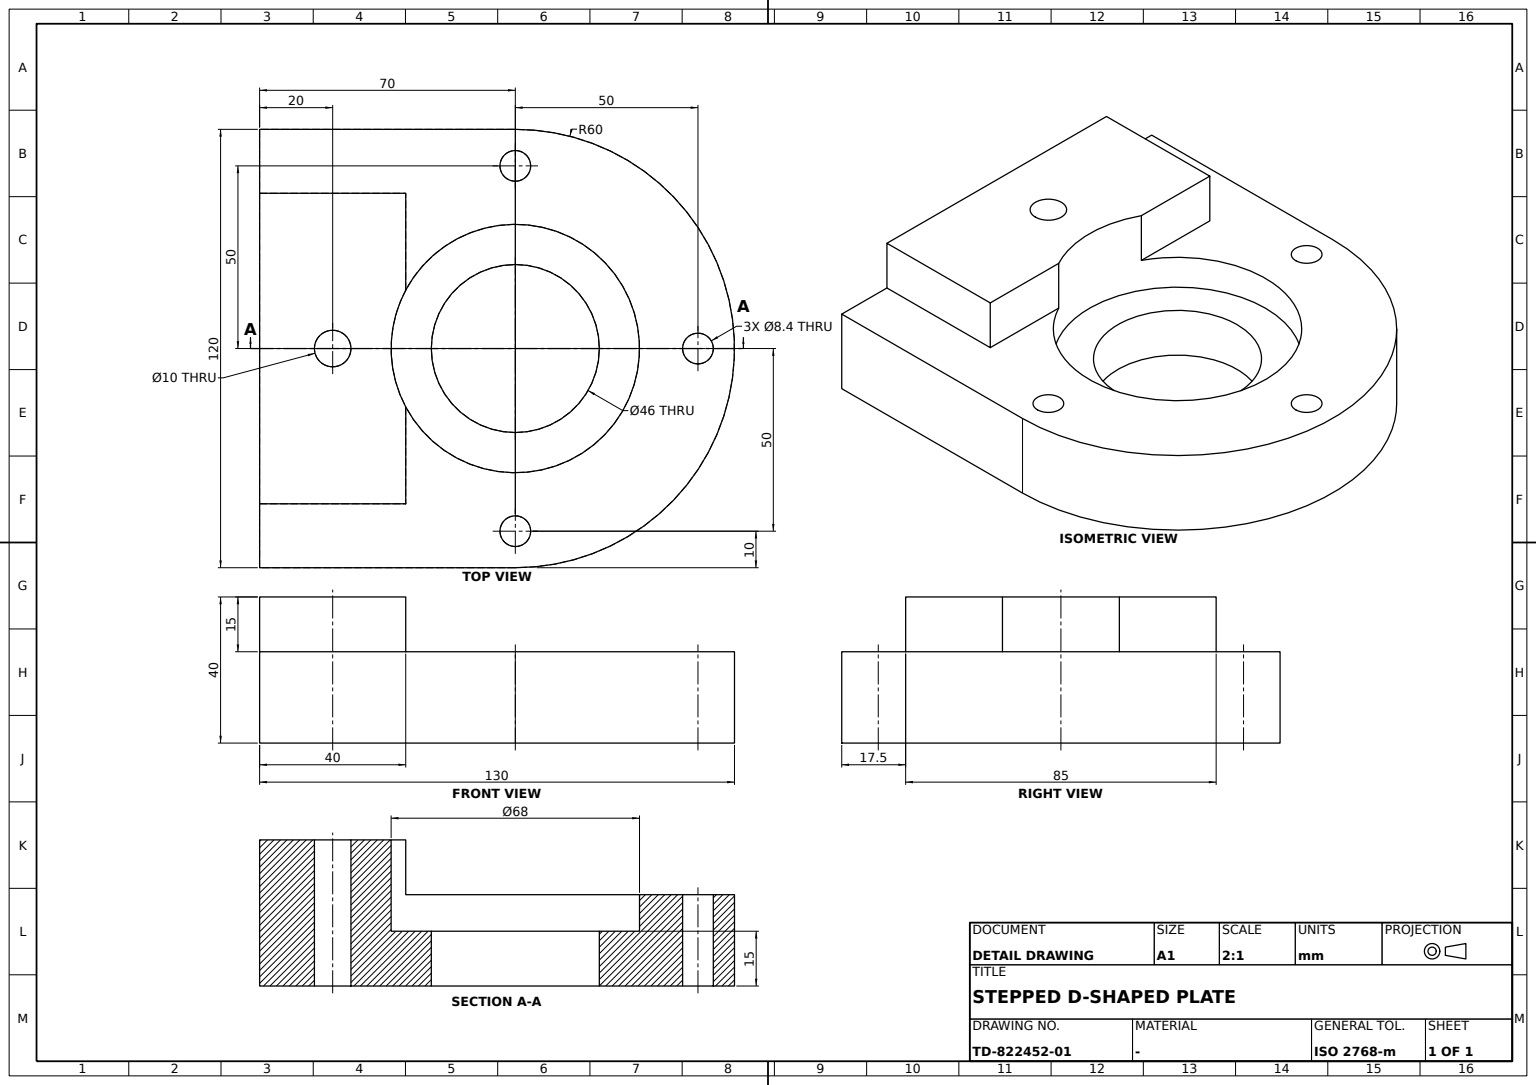
ISO-10303-21;
HEADER;
FILE_DESCRIPTION((''),'2;1');
FILE_NAME('','',(''),(''),'','','');
FILE_SCHEMA(('AUTOMOTIVE_DESIGN'));
ENDSEC;
DATA;
#1=APPLICATION_CONTEXT('');
#2=PRODUCT_CONTEXT('',#1,'mechanical');
#3=PRODUCT('','','',(#2));
#4=PRODUCT_DEFINITION_FORMATION('','',#3);
#5=PRODUCT_DEFINITION_CONTEXT('',#1,'design');
#6=PRODUCT_DEFINITION('','',#4,#5);
#7=PRODUCT_DEFINITION_SHAPE('','',#6);
#8=(LENGTH_UNIT()NAMED_UNIT(*)SI_UNIT(.MILLI.,.METRE.));
#9=(NAMED_UNIT(*)PLANE_ANGLE_UNIT()SI_UNIT($,.RADIAN.));
#10=(NAMED_UNIT(*)SI_UNIT($,.STERADIAN.)SOLID_ANGLE_UNIT());
#11=UNCERTAINTY_MEASURE_WITH_UNIT(LENGTH_MEASURE(0.005),#8,'distance_accuracy_value','');
#12=(GEOMETRIC_REPRESENTATION_CONTEXT(3)GLOBAL_UNCERTAINTY_ASSIGNED_CONTEXT((#11))GLOBAL_UNIT_ASSIGNED_CONTEXT((#8,#9,#10))REPRESENTATION_CONTEXT('',''));
#13=CARTESIAN_POINT('',(-45.797717,0.,25.));
#14=VERTEX_POINT('',#13);
#15=CARTESIAN_POINT('',(-50.,0.,25.));
#16=DIRECTION('',(0.,0.,1.));
#17=DIRECTION('',(1.,0.,0.));
#18=AXIS2_PLACEMENT_3D('',#15,#16,#17);
#19=CIRCLE('',#18,4.202283);
#20=EDGE_CURVE('',#14,#14,#19,.T.);
#21=ORIENTED_EDGE('',*,*,#20,.T.);
#22=EDGE_LOOP('',(#21));
#23=FACE_BOUND('',#22,.T.);
#24=CARTESIAN_POINT('',(-45.797717,0.,0.));
#25=VERTEX_POINT('',#24);
#26=CARTESIAN_POINT('',(-50.,0.,0.));
#27=AXIS2_PLACEMENT_3D('',#26,#16,#17);
#28=CIRCLE('',#27,4.202283);
#29=EDGE_CURVE('',#25,#25,#28,.T.);
#30=ORIENTED_EDGE('',*,*,#29,.F.);
#31=EDGE_LOOP('',(#30));
#32=FACE_BOUND('',#31,.T.);
#33=CARTESIAN_POINT('',(-50.,0.,11.84));
#34=DIRECTION('',(0.,1.,0.));
#35=AXIS2_PLACEMENT_3D('',#33,#16,#34);
#36=CYLINDRICAL_SURFACE('',#35,4.202283);
#37=ADVANCED_FACE('',(#23,#32),#36,.F.);
#38=CARTESIAN_POINT('',(-16.,-30.,25.));
#39=VERTEX_POINT('',#38);
#40=CARTESIAN_POINT('',(-16.,-30.,40.));
#41=VERTEX_POINT('',#40);
#42=DIRECTION('',(0.,0.,-1.));
#43=VECTOR('',#42,1000.);
#44=LINE('',#38,#43);
#45=EDGE_CURVE('',#39,#41,#44,.F.);
#46=ORIENTED_EDGE('',*,*,#45,.F.);
#47=CARTESIAN_POINT('',(-42.5,-30.,25.));
#48=VERTEX_POINT('',#47);
#49=CARTESIAN_POINT('',(0.,-30.,25.));
#50=DIRECTION('',(-1.,0.,0.));
#51=VECTOR('',#50,1000.);
#52=LINE('',#49,#51);
#53=EDGE_CURVE('',#39,#48,#52,.T.);
#54=ORIENTED_EDGE('',*,*,#53,.T.);
#55=CARTESIAN_POINT('',(-42.5,-30.,40.));
#56=VERTEX_POINT('',#55);
#57=VECTOR('',#16,1000.);
#58=LINE('',#47,#57);
#59=EDGE_CURVE('',#48,#56,#58,.T.);
#60=ORIENTED_EDGE('',*,*,#59,.T.);
#61=CARTESIAN_POINT('',(0.,-30.,40.));
#62=LINE('',#61,#51);
#63=EDGE_CURVE('',#41,#56,#62,.T.);
#64=ORIENTED_EDGE('',*,*,#63,.F.);
#65=EDGE_LOOP('',(#46,#54,#60,#64));
#66=FACE_BOUND('',#65,.T.);
#67=CARTESIAN_POINT('',(42.5,-30.,25.));
#68=AXIS2_PLACEMENT_3D('',#67,#34,#50);
#69=PLANE('',#68);
#70=ADVANCED_FACE('',(#66),#69,.T.);
#71=CARTESIAN_POINT('',(-34.,0.,15.));
#72=VERTEX_POINT('',#71);
#73=CARTESIAN_POINT('',(0.,0.,15.));
#74=AXIS2_PLACEMENT_3D('',#73,#42,#50);
#75=CIRCLE('',#74,34.);
#76=EDGE_CURVE('',#72,#72,#75,.T.);
#77=ORIENTED_EDGE('',*,*,#76,.F.);
#78=EDGE_LOOP('',(#77));
#79=FACE_BOUND('',#78,.T.);
#80=CARTESIAN_POINT('',(-23.,0.,15.));
#81=VERTEX_POINT('',#80);
#82=CIRCLE('',#74,23.);
#83=EDGE_CURVE('',#81,#81,#82,.T.);
#84=ORIENTED_EDGE('',*,*,#83,.T.);
#85=EDGE_LOOP('',(#84));
#86=FACE_BOUND('',#85,.T.);
#87=AXIS2_PLACEMENT_3D('',#73,#42,#17);
#88=PLANE('',#87);
#89=ADVANCED_FACE('',(#79,#86),#88,.F.);
#90=CARTESIAN_POINT('',(-60.,0.,0.));
#91=VERTEX_POINT('',#90);
#92=CARTESIAN_POINT('',(-60.,0.,25.));
#93=VERTEX_POINT('',#92);
#94=CARTESIAN_POINT('',(-60.,0.,12.5));
#95=LINE('',#94,#57);
#96=EDGE_CURVE('',#91,#93,#95,.T.);
#97=ORIENTED_EDGE('',*,*,#96,.T.);
#98=CARTESIAN_POINT('',(60.,0.,25.));
#99=VERTEX_POINT('',#98);
#100=CARTESIAN_POINT('',(0.,0.,25.));
#101=AXIS2_PLACEMENT_3D('',#100,#16,#17);
#102=CIRCLE('',#101,60.);
#103=EDGE_CURVE('',#99,#93,#102,.T.);
#104=ORIENTED_EDGE('',*,*,#103,.F.);
#105=CARTESIAN_POINT('',(60.,0.,0.));
#106=VERTEX_POINT('',#105);
#107=CARTESIAN_POINT('',(60.,0.,12.5));
#108=LINE('',#107,#57);
#109=EDGE_CURVE('',#106,#99,#108,.T.);
#110=ORIENTED_EDGE('',*,*,#109,.F.);
#111=CARTESIAN_POINT('',(0.,0.,0.));
#112=AXIS2_PLACEMENT_3D('',#111,#16,#17);
#113=CIRCLE('',#112,60.);
#114=EDGE_CURVE('',#106,#91,#113,.T.);
#115=ORIENTED_EDGE('',*,*,#114,.T.);
#116=EDGE_LOOP('',(#97,#104,#110,#115));
#117=FACE_BOUND('',#116,.T.);
#118=CARTESIAN_POINT('',(0.,0.,12.5));
#119=AXIS2_PLACEMENT_3D('',#118,#16,#34);
#120=CYLINDRICAL_SURFACE('',#119,60.);
#121=ADVANCED_FACE('',(#117),#120,.T.);
#122=CARTESIAN_POINT('',(-60.,-70.,0.));
#123=VERTEX_POINT('',#122);
#124=CARTESIAN_POINT('',(-60.,-70.,25.));
#125=VERTEX_POINT('',#124);
#126=LINE('',#122,#57);
#127=EDGE_CURVE('',#123,#125,#126,.T.);
#128=ORIENTED_EDGE('',*,*,#127,.T.);
#129=DIRECTION('',(0.,-1.,0.));
#130=VECTOR('',#129,1000.);
#131=LINE('',#92,#130);
#132=EDGE_CURVE('',#93,#125,#131,.T.);
#133=ORIENTED_EDGE('',*,*,#132,.F.);
#134=ORIENTED_EDGE('',*,*,#96,.F.);
#135=LINE('',#90,#130);
#136=EDGE_CURVE('',#91,#123,#135,.T.);
#137=ORIENTED_EDGE('',*,*,#136,.T.);
#138=EDGE_LOOP('',(#128,#133,#134,#137));
#139=FACE_BOUND('',#138,.T.);
#140=AXIS2_PLACEMENT_3D('',#90,#50,#129);
#141=PLANE('',#140);
#142=ADVANCED_FACE('',(#139),#141,.T.);
#143=CARTESIAN_POINT('',(-42.5,-70.,25.));
#144=VERTEX_POINT('',#143);
#145=CARTESIAN_POINT('',(0.,-70.,25.));
#146=VECTOR('',#17,1000.);
#147=LINE('',#145,#146);
#148=EDGE_CURVE('',#125,#144,#147,.T.);
#149=ORIENTED_EDGE('',*,*,#148,.F.);
#150=ORIENTED_EDGE('',*,*,#127,.F.);
#151=CARTESIAN_POINT('',(60.,-70.,0.));
#152=VERTEX_POINT('',#151);
#153=CARTESIAN_POINT('',(0.,-70.,0.));
#154=LINE('',#153,#146);
#155=EDGE_CURVE('',#123,#152,#154,.T.);
#156=ORIENTED_EDGE('',*,*,#155,.T.);
#157=CARTESIAN_POINT('',(60.,-70.,25.));
#158=VERTEX_POINT('',#157);
#159=LINE('',#151,#57);
#160=EDGE_CURVE('',#152,#158,#159,.T.);
#161=ORIENTED_EDGE('',*,*,#160,.T.);
#162=CARTESIAN_POINT('',(42.5,-70.,25.));
#163=VERTEX_POINT('',#162);
#164=EDGE_CURVE('',#163,#158,#147,.T.);
#165=ORIENTED_EDGE('',*,*,#164,.F.);
#166=CARTESIAN_POINT('',(42.5,-70.,40.));
#167=VERTEX_POINT('',#166);
#168=LINE('',#162,#57);
#169=EDGE_CURVE('',#163,#167,#168,.T.);
#170=ORIENTED_EDGE('',*,*,#169,.T.);
#171=CARTESIAN_POINT('',(-42.5,-70.,40.));
#172=VERTEX_POINT('',#171);
#173=CARTESIAN_POINT('',(0.,-70.,40.));
#174=LINE('',#173,#146);
#175=EDGE_CURVE('',#172,#167,#174,.T.);
#176=ORIENTED_EDGE('',*,*,#175,.F.);
#177=CARTESIAN_POINT('',(-42.5,-70.,0.));
#178=LINE('',#177,#57);
#179=EDGE_CURVE('',#144,#172,#178,.T.);
#180=ORIENTED_EDGE('',*,*,#179,.F.);
#181=EDGE_LOOP('',(#149,#150,#156,#161,#165,#170,#176,#180));
#182=FACE_BOUND('',#181,.T.);
#183=AXIS2_PLACEMENT_3D('',#122,#129,#17);
#184=PLANE('',#183);
#185=ADVANCED_FACE('',(#182),#184,.T.);
#186=ORIENTED_EDGE('',*,*,#169,.F.);
#187=VERTEX_POINT('',#67);
#188=CARTESIAN_POINT('',(42.5,0.,25.));
#189=LINE('',#188,#130);
#190=EDGE_CURVE('',#187,#163,#189,.T.);
#191=ORIENTED_EDGE('',*,*,#190,.F.);
#192=CARTESIAN_POINT('',(42.5,-30.,40.));
#193=VERTEX_POINT('',#192);
#194=LINE('',#67,#57);
#195=EDGE_CURVE('',#187,#193,#194,.T.);
#196=ORIENTED_EDGE('',*,*,#195,.T.);
#197=CARTESIAN_POINT('',(42.5,0.,40.));
#198=LINE('',#197,#130);
#199=EDGE_CURVE('',#193,#167,#198,.T.);
#200=ORIENTED_EDGE('',*,*,#199,.T.);
#201=EDGE_LOOP('',(#186,#191,#196,#200));
#202=FACE_BOUND('',#201,.T.);
#203=AXIS2_PLACEMENT_3D('',#67,#50,#129);
#204=PLANE('',#203);
#205=ADVANCED_FACE('',(#202),#204,.F.);
#206=CARTESIAN_POINT('',(4.202283,50.,25.));
#207=VERTEX_POINT('',#206);
#208=CARTESIAN_POINT('',(0.,50.,25.));
#209=AXIS2_PLACEMENT_3D('',#208,#16,#17);
#210=CIRCLE('',#209,4.202283);
#211=EDGE_CURVE('',#207,#207,#210,.T.);
#212=ORIENTED_EDGE('',*,*,#211,.F.);
#213=EDGE_LOOP('',(#212));
#214=FACE_BOUND('',#213,.T.);
#215=ORIENTED_EDGE('',*,*,#148,.T.);
#216=CARTESIAN_POINT('',(-42.5,0.,25.));
#217=VECTOR('',#34,1000.);
#218=LINE('',#216,#217);
#219=EDGE_CURVE('',#144,#48,#218,.T.);
#220=ORIENTED_EDGE('',*,*,#219,.T.);
#221=ORIENTED_EDGE('',*,*,#53,.F.);
#222=CARTESIAN_POINT('',(16.,-30.,25.));
#223=VERTEX_POINT('',#222);
#224=CIRCLE('',#101,34.);
#225=EDGE_CURVE('',#223,#39,#224,.T.);
#226=ORIENTED_EDGE('',*,*,#225,.F.);
#227=EDGE_CURVE('',#187,#223,#52,.T.);
#228=ORIENTED_EDGE('',*,*,#227,.F.);
#229=ORIENTED_EDGE('',*,*,#190,.T.);
#230=ORIENTED_EDGE('',*,*,#164,.T.);
#231=LINE('',#98,#130);
#232=EDGE_CURVE('',#99,#158,#231,.T.);
#233=ORIENTED_EDGE('',*,*,#232,.F.);
#234=ORIENTED_EDGE('',*,*,#103,.T.);
#235=ORIENTED_EDGE('',*,*,#132,.T.);
#236=EDGE_LOOP('',(#215,#220,#221,#226,#228,#229,#230,#233,#234,#235));
#237=FACE_BOUND('',#236,.T.);
#238=ORIENTED_EDGE('',*,*,#20,.F.);
#239=EDGE_LOOP('',(#238));
#240=FACE_BOUND('',#239,.T.);
#241=CARTESIAN_POINT('',(54.202283,0.,25.));
#242=VERTEX_POINT('',#241);
#243=CARTESIAN_POINT('',(50.,0.,25.));
#244=AXIS2_PLACEMENT_3D('',#243,#16,#17);
#245=CIRCLE('',#244,4.202283);
#246=EDGE_CURVE('',#242,#242,#245,.T.);
#247=ORIENTED_EDGE('',*,*,#246,.F.);
#248=EDGE_LOOP('',(#247));
#249=FACE_BOUND('',#248,.T.);
#250=AXIS2_PLACEMENT_3D('',#100,#16,#34);
#251=PLANE('',#250);
#252=ADVANCED_FACE('',(#214,#237,#240,#249),#251,.T.);
#253=ORIENTED_EDGE('',*,*,#83,.F.);
#254=EDGE_LOOP('',(#253));
#255=FACE_BOUND('',#254,.T.);
#256=CARTESIAN_POINT('',(23.,0.,0.));
#257=VERTEX_POINT('',#256);
#258=CIRCLE('',#112,23.);
#259=EDGE_CURVE('',#257,#257,#258,.T.);
#260=ORIENTED_EDGE('',*,*,#259,.F.);
#261=EDGE_LOOP('',(#260));
#262=FACE_BOUND('',#261,.T.);
#263=CARTESIAN_POINT('',(0.,0.,14.9));
#264=AXIS2_PLACEMENT_3D('',#263,#42,#17);
#265=CYLINDRICAL_SURFACE('',#264,23.);
#266=ADVANCED_FACE('',(#255,#262),#265,.F.);
#267=ORIENTED_EDGE('',*,*,#246,.T.);
#268=EDGE_LOOP('',(#267));
#269=FACE_BOUND('',#268,.T.);
#270=CARTESIAN_POINT('',(54.202283,0.,0.));
#271=VERTEX_POINT('',#270);
#272=CARTESIAN_POINT('',(50.,0.,0.));
#273=AXIS2_PLACEMENT_3D('',#272,#16,#17);
#274=CIRCLE('',#273,4.202283);
#275=EDGE_CURVE('',#271,#271,#274,.T.);
#276=ORIENTED_EDGE('',*,*,#275,.F.);
#277=EDGE_LOOP('',(#276));
#278=FACE_BOUND('',#277,.T.);
#279=CARTESIAN_POINT('',(50.,0.,11.84));
#280=AXIS2_PLACEMENT_3D('',#279,#16,#34);
#281=CYLINDRICAL_SURFACE('',#280,4.202283);
#282=ADVANCED_FACE('',(#269,#278),#281,.F.);
#283=ORIENTED_EDGE('',*,*,#29,.T.);
#284=EDGE_LOOP('',(#283));
#285=FACE_BOUND('',#284,.T.);
#286=LINE('',#105,#130);
#287=EDGE_CURVE('',#106,#152,#286,.T.);
#288=ORIENTED_EDGE('',*,*,#287,.T.);
#289=ORIENTED_EDGE('',*,*,#155,.F.);
#290=ORIENTED_EDGE('',*,*,#136,.F.);
#291=ORIENTED_EDGE('',*,*,#114,.F.);
#292=EDGE_LOOP('',(#288,#289,#290,#291));
#293=FACE_BOUND('',#292,.T.);
#294=CARTESIAN_POINT('',(5.,-50.,0.));
#295=VERTEX_POINT('',#294);
#296=CARTESIAN_POINT('',(0.,-50.,0.));
#297=AXIS2_PLACEMENT_3D('',#296,#16,#17);
#298=CIRCLE('',#297,5.);
#299=EDGE_CURVE('',#295,#295,#298,.T.);
#300=ORIENTED_EDGE('',*,*,#299,.T.);
#301=EDGE_LOOP('',(#300));
#302=FACE_BOUND('',#301,.T.);
#303=ORIENTED_EDGE('',*,*,#259,.T.);
#304=EDGE_LOOP('',(#303));
#305=FACE_BOUND('',#304,.T.);
#306=CARTESIAN_POINT('',(4.202283,50.,0.));
#307=VERTEX_POINT('',#306);
#308=CARTESIAN_POINT('',(0.,50.,0.));
#309=AXIS2_PLACEMENT_3D('',#308,#16,#17);
#310=CIRCLE('',#309,4.202283);
#311=EDGE_CURVE('',#307,#307,#310,.T.);
#312=ORIENTED_EDGE('',*,*,#311,.T.);
#313=EDGE_LOOP('',(#312));
#314=FACE_BOUND('',#313,.T.);
#315=ORIENTED_EDGE('',*,*,#275,.T.);
#316=EDGE_LOOP('',(#315));
#317=FACE_BOUND('',#316,.T.);
#318=AXIS2_PLACEMENT_3D('',#111,#16,#34);
#319=PLANE('',#318);
#320=ADVANCED_FACE('',(#285,#293,#302,#305,#314,#317),#319,.F.);
#321=ORIENTED_EDGE('',*,*,#299,.F.);
#322=EDGE_LOOP('',(#321));
#323=FACE_BOUND('',#322,.T.);
#324=CARTESIAN_POINT('',(5.,-50.,40.));
#325=VERTEX_POINT('',#324);
#326=CARTESIAN_POINT('',(0.,-50.,40.));
#327=AXIS2_PLACEMENT_3D('',#326,#16,#17);
#328=CIRCLE('',#327,5.);
#329=EDGE_CURVE('',#325,#325,#328,.T.);
#330=ORIENTED_EDGE('',*,*,#329,.T.);
#331=EDGE_LOOP('',(#330));
#332=FACE_BOUND('',#331,.T.);
#333=CARTESIAN_POINT('',(0.,-50.,19.34));
#334=AXIS2_PLACEMENT_3D('',#333,#16,#34);
#335=CYLINDRICAL_SURFACE('',#334,5.);
#336=ADVANCED_FACE('',(#323,#332),#335,.F.);
#337=ORIENTED_EDGE('',*,*,#311,.F.);
#338=EDGE_LOOP('',(#337));
#339=FACE_BOUND('',#338,.T.);
#340=ORIENTED_EDGE('',*,*,#211,.T.);
#341=EDGE_LOOP('',(#340));
#342=FACE_BOUND('',#341,.T.);
#343=CARTESIAN_POINT('',(0.,50.,11.84));
#344=AXIS2_PLACEMENT_3D('',#343,#16,#34);
#345=CYLINDRICAL_SURFACE('',#344,4.202283);
#346=ADVANCED_FACE('',(#339,#342),#345,.F.);
#347=CARTESIAN_POINT('',(16.,-30.,40.));
#348=VERTEX_POINT('',#347);
#349=LINE('',#222,#43);
#350=EDGE_CURVE('',#348,#223,#349,.T.);
#351=ORIENTED_EDGE('',*,*,#350,.F.);
#352=EDGE_CURVE('',#193,#348,#62,.T.);
#353=ORIENTED_EDGE('',*,*,#352,.F.);
#354=ORIENTED_EDGE('',*,*,#195,.F.);
#355=ORIENTED_EDGE('',*,*,#227,.T.);
#356=EDGE_LOOP('',(#351,#353,#354,#355));
#357=FACE_BOUND('',#356,.T.);
#358=ADVANCED_FACE('',(#357),#69,.T.);
#359=ORIENTED_EDGE('',*,*,#76,.T.);
#360=EDGE_LOOP('',(#359));
#361=FACE_BOUND('',#360,.T.);
#362=CARTESIAN_POINT('',(0.,0.,40.));
#363=AXIS2_PLACEMENT_3D('',#362,#16,#17);
#364=CIRCLE('',#363,34.);
#365=EDGE_CURVE('',#41,#348,#364,.T.);
#366=ORIENTED_EDGE('',*,*,#365,.T.);
#367=ORIENTED_EDGE('',*,*,#350,.T.);
#368=ORIENTED_EDGE('',*,*,#225,.T.);
#369=ORIENTED_EDGE('',*,*,#45,.T.);
#370=EDGE_LOOP('',(#366,#367,#368,#369));
#371=FACE_BOUND('',#370,.T.);
#372=CARTESIAN_POINT('',(0.,0.,24.9));
#373=AXIS2_PLACEMENT_3D('',#372,#42,#17);
#374=CYLINDRICAL_SURFACE('',#373,34.);
#375=ADVANCED_FACE('',(#361,#371),#374,.F.);
#376=ORIENTED_EDGE('',*,*,#199,.F.);
#377=ORIENTED_EDGE('',*,*,#352,.T.);
#378=ORIENTED_EDGE('',*,*,#365,.F.);
#379=ORIENTED_EDGE('',*,*,#63,.T.);
#380=CARTESIAN_POINT('',(-42.5,0.,40.));
#381=LINE('',#380,#217);
#382=EDGE_CURVE('',#172,#56,#381,.T.);
#383=ORIENTED_EDGE('',*,*,#382,.F.);
#384=ORIENTED_EDGE('',*,*,#175,.T.);
#385=EDGE_LOOP('',(#376,#377,#378,#379,#383,#384));
#386=FACE_BOUND('',#385,.T.);
#387=ORIENTED_EDGE('',*,*,#329,.F.);
#388=EDGE_LOOP('',(#387));
#389=FACE_BOUND('',#388,.T.);
#390=AXIS2_PLACEMENT_3D('',#362,#16,#34);
#391=PLANE('',#390);
#392=ADVANCED_FACE('',(#386,#389),#391,.T.);
#393=ORIENTED_EDGE('',*,*,#59,.F.);
#394=ORIENTED_EDGE('',*,*,#219,.F.);
#395=ORIENTED_EDGE('',*,*,#179,.T.);
#396=ORIENTED_EDGE('',*,*,#382,.T.);
#397=EDGE_LOOP('',(#393,#394,#395,#396));
#398=FACE_BOUND('',#397,.T.);
#399=AXIS2_PLACEMENT_3D('',#143,#17,#34);
#400=PLANE('',#399);
#401=ADVANCED_FACE('',(#398),#400,.F.);
#402=ORIENTED_EDGE('',*,*,#160,.F.);
#403=ORIENTED_EDGE('',*,*,#287,.F.);
#404=ORIENTED_EDGE('',*,*,#109,.T.);
#405=ORIENTED_EDGE('',*,*,#232,.T.);
#406=EDGE_LOOP('',(#402,#403,#404,#405));
#407=FACE_BOUND('',#406,.T.);
#408=AXIS2_PLACEMENT_3D('',#105,#50,#129);
#409=PLANE('',#408);
#410=ADVANCED_FACE('',(#407),#409,.F.);
#411=CLOSED_SHELL('',(#37,#70,#89,#121,#142,#185,#205,#252,#266,#282,#320,#336,#346,#358,#375,#392,#401,#410));
#412=MANIFOLD_SOLID_BREP('',#411);
#413=ADVANCED_BREP_SHAPE_REPRESENTATION('',(#412),#12);
#414=SHAPE_DEFINITION_REPRESENTATION(#7,#413);
ENDSEC;
END-ISO-10303-21;
